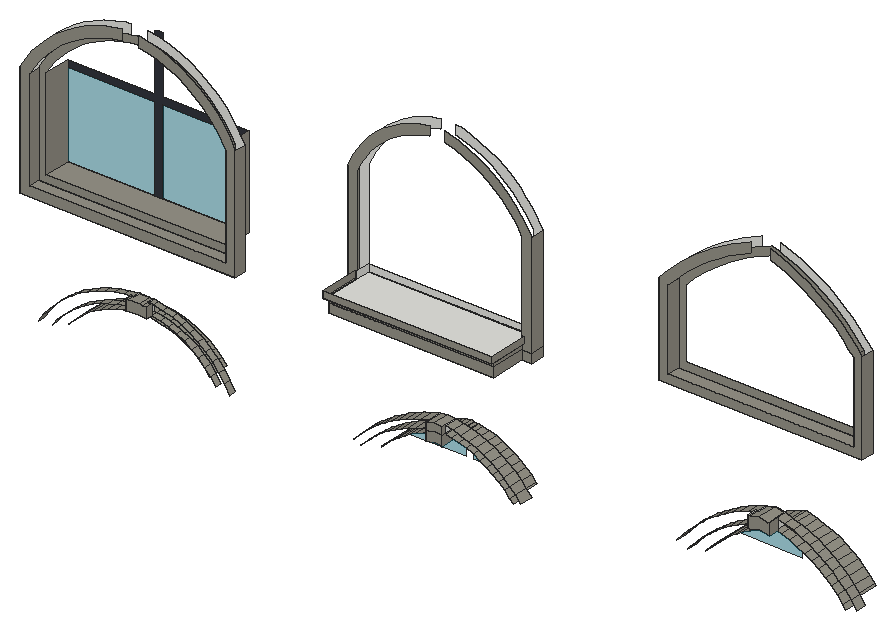
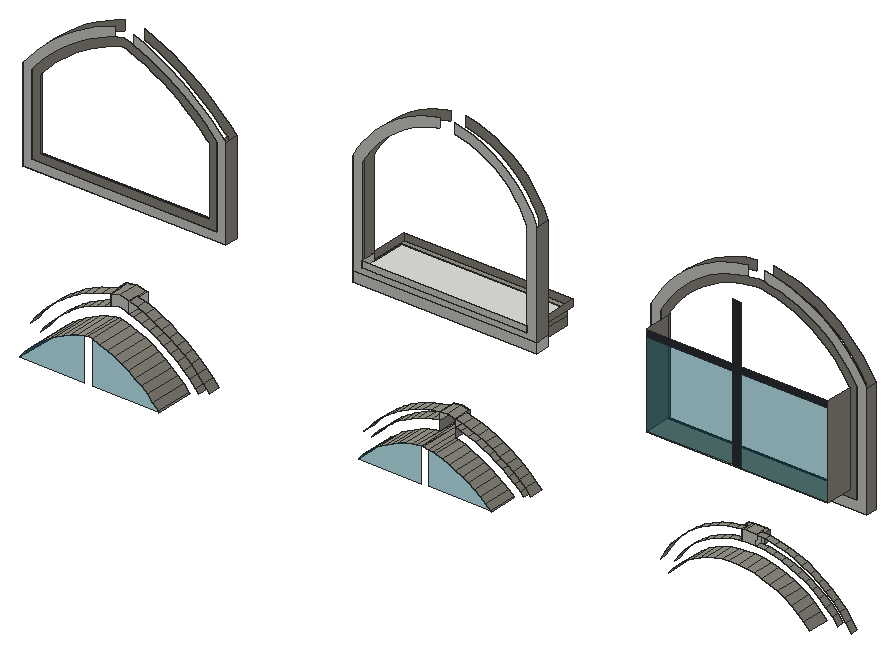
# SketchUp Ruby script. Lengths in inches.
U = 1.inch
M = Sketchup.active_model
def pt(a) = Geom::Point3d.new(a.map { |v| v * U })
def face(e, loops, mat)
  f = e.add_face(loops[0].map { |a| pt(a) })
  loops[1..].each { |l| e.add_face(l.map { |a| pt(a) }).erase! }
  f.material = f.back_material = mat if mat
  f
end
# faces: each face lists its corners as indices into pts; further lists are holes
def faces(e, pts, list, mat = nil) = list.each { |f| face(e, (f[0].is_a?(Array) ? f : [f]).map { |l| l.map { |i| pts[i] } }, mat) }
# xy, xz, yz: faces in a plane at the given z, y or x. An outline is a flat list of corners, or four numbers for a rectangle; further outlines are holes
def ring(l) = l.size == 4 ? [[l[0], l[1]], [l[2], l[1]], [l[2], l[3]], [l[0], l[3]]] : l.each_slice(2).to_a
def flat(e, list, mat, &to3) = list.each { |f| face(e, (f[0].is_a?(Array) ? f : [f]).map { |l| ring(l).map { |u, v| to3.(u, v) } }, mat) }
def xy(e, z, list, mat = nil) = flat(e, list, mat) { |x, y| [x, y, z] }
def xz(e, y, list, mat = nil) = flat(e, list, mat) { |x, z| [x, y, z] }
def yz(e, x, list, mat = nil) = flat(e, list, mat) { |y, z| [x, y, z] }
def lines(e, pts, list) = list.each { |a, b| e.add_line(pt(pts[a]), pt(pts[b])) }
# prism: a flat outline (further loops are holes) pulled along v
def prism(e, loops, v, mat = nil)
  f = face(e, loops, mat); d = Geom::Vector3d.new(v.map { |x| x * U })
  f.pushpull(f.normal.samedirection?(d) ? d.length : -d.length)
end
def box(e, o, s, mat = nil) = prism(e, [[o, [o[0] + s[0], o[1], o[2]], [o[0] + s[0], o[1] + s[1], o[2]], [o[0], o[1] + s[1], o[2]]]], [0, 0, s[2]], mat)
def at(x, y, z, deg = 0) = Geom::Transformation.translation(pt([x, y, z])) * Geom::Transformation.rotation(ORIGIN, Z_AXIS, deg.degrees)
def axes(o, x, y, z) = Geom::Transformation.new([*x, 0, *y, 0, *z, 0, *pt(o).to_a, 1])
def part(name) = M.definitions.add(name)
# library, detail: a bought-in or finely detailed component or shape, given as its bounding box
def library(name, o, s) = part(name).tap { |d| box(d.entities, o, s) }
def detail(e, o, s) = box(e.add_group.entities, o, s)
def put(e, d, t, mat = nil) = e.add_instance(d, t).tap { |i| i.material = mat if mat }
def group(e, t, mat = nil) = e.add_group.tap { |g| g.transformation = t; g.material = mat if mat }.entities
root = M.entities
M.materials.add("[Formica Graystone]").color = [149, 146, 135]
M.materials.add("[Formica Laminate Dark]").color = [50, 53, 60]
M.materials.add("[Translucent Glass Tinted]").color = [4, 106, 127]
M.materials["[Translucent Glass Tinted]"].alpha = 0.48
xy(root,272.42,[[104.39,144.04,108.99,154.66]],"[Formica Graystone]")
xy(root,276.05,[[111.06,137.54,112.68,140.72]],"[Formica Graystone]")
xy(root,276.22,[[104.21,137.54,109.15,144.04]],"[Formica Graystone]")
xy(root,280.43,[[405.62,147.86,406.74,152.99]],"[Formica Graystone]")
xy(root,280.76,[[415.58,147.86,416.39,152.99]],"[Formica Graystone]")
xy(root,281.33,[[111.06,137.54,112.68,140.72]],"[Formica Graystone]")
xy(root,281.47,[[103.95,137.54,109.38,144.04]],"[Formica Graystone]")
xy(root,286.13,[[405.62,147.86,406.74,152.99]],"[Formica Graystone]")
xy(root,286.38,[[415.58,147.86,416.39,152.99]],"[Formica Graystone]")
xy(root,309.5625,[[48.72,138.29,156.59,144.04]])
xy(root,314.51,[[53.67,138.29,151.64,144.04]],"[Formica Graystone]")
xy(root,318.06,[[57.22,144.04,148.1,157.6]],"[Formica Graystone]")
xy(root,323.85,[[218.68,119.22,218.68,136.91,213.99,136.91,213.99,144.04,306.11,144.04,306.11,136.91,301.43,136.91,301.43,119.22]],"[Formica Graystone]")
xy(root,328.26,[[358.05,151.8,459.74,158.3]],"[Formica Graystone]")
xy(root,328.54,[[218.68,119.22,301.43,119.22,301.43,136.91,306.11,136.91,306.11,144.04,213.99,144.04,213.99,136.91,218.68,136.91]])
xy(root,331.48,[[218.68,119.22,301.43,144.04]])
xy(root,331.48,[[217.8,116.35,218.68,136.91],[218.68,116.35,302.43,119.22],[301.43,119.22,302.43,136.91]],"[Formica Graystone]")
xy(root,332.71,[[362.5,151.8,455.3,158.3]],"[Formica Graystone]")
xz(root,116.35,[[217.8,331.48,302.43,334.79]],"[Formica Graystone]")
xz(root,119.22,[[218.68,323.85,301.43,328.54],[218.68,328.54,301.43,331.48]],"[Formica Graystone]")
xz(root,135.35,[[254.54,271.77,256.47,272.28,258.86,272.77,261.26,272.49,262.53,272.25,262.53,277.12,261.98,277.22,258.65,277.61,255.38,276.9375,254.54,276.72],[254.54,276.72,255.38,276.9375,258.65,277.61,261.98,277.22,262.53,277.12,262.53,280.87,258.49,281.34,254.54,280.53]],"[Formica Graystone]")
xz(root,136.91,[[217.8,331.48,218.68,334.79],[301.43,331.48,302.43,334.79]])
xz(root,136.91,[[213.99,323.85,218.68,328.54],[301.43,323.85,306.11,328.54],[213.99,328.54,218.68,328.54,218.68,331.48,217.8,331.48,217.8,334.79,218.68,334.79,218.68,379.39,220.23,382.79,222.51,386.72,225.14,390.41,228.11,393.84,231.39,396.98,234.95,399.79,238.76,402.25,242.79,404.34,246.99,406.05,251.34,407.34,255.1,408.09,255.1,412.87,250.21,411.9,245.4375,410.47,240.82,408.6,236.4,406.31,232.22,403.6,228.31,400.52,224.71,397.08,221.45,393.3125,218.56,389.25,216.07,384.94,213.99,380.42],[301.43,328.54,306.11,328.54,306.11,380.42,303.62,384.61,300.82,388.61,297.72,392.39,294.35,395.92,290.73,399.19,286.86,402.18,282.79,404.87,278.52,407.25,274.09,409.29,269.52,411,264.83,412.37,262.44,412.87,262.44,408.08,263.69,407.82,268.04,406.55,272.29,404.97,276.4,403.07,280.36,400.86,284.14,398.37,287.72,395.59,291.08,392.56,294.21,389.28,297.08,385.78,299.68,382.07,301.43,379.13,301.43,334.79,302.43,334.79,302.43,331.48,301.43,331.48]],"[Formica Graystone]")
xz(root,137.54,[[111.06,276.05,112.68,276.05,112.68,281.33,111.06,281.33,109.38,281.47,103.95,281.47,102.33,281.4,102.59,276.14,104.21,276.22,109.15,276.22]],"[Formica Graystone]")
xz(root,138.29,[[48.72,309.5625,156.59,309.5625,156.59,366.1875,153.85,371.09,150.69,375.74,147.13,380.09,143.21,384.11,138.94,387.77,134.375,391.05,129.53,393.91,124.46,396.33,119.2,398.3,113.78,399.8,108.25,400.8125,108.25,395.78,112.67,394.96,117.67,393.58,122.52,391.77,127.2,389.53,131.67,386.89,135.88,383.875,139.82,380.5,143.4375,376.79,146.72,372.77,149.64,368.49,151.64,364.9,151.64,314.51,53.67,314.51,53.67,364.79,55.75,368.18,58.81,372.37,62.1875,376.29,65.875,379.93,69.84,383.26,74.0625,386.26,78.51,388.91,83.16,391.19,87.98,393.1,92.93,394.6,97.99,395.71,99.89,395.97,99.89,400.96,97.13,400.59,91.68,399.4,86.34,397.78,81.15,395.73,76.15,393.27,71.35,390.41,66.81,387.18,62.54,383.59,58.57,379.67,54.92,375.45,51.64,370.94,48.72,366.1875]],"[Formica Graystone]")
xz(root,140.72,[[111.06,276.05,112.68,276.05,112.68,281.1875,111.06,281.33],[102.59,276.14,104.21,276.22,103.95,281.47,102.33,281.32],[112.68,281.1875,111.06,281.33,112.68,281.33],[102.33,281.32,102.33,281.4,103.95,281.47]])
xz(root,144.04,[[111.06,276.05,109.15,276.22,104.21,276.22,103.95,281.47,109.38,281.47,111.06,281.33],[103.95,281.47,109.38,281.47,108.82,281.52],[48.72,309.5625,48.72,366.1875,51.64,370.94,54.92,375.45,58.57,379.67,62.54,383.59,66.81,387.18,71.35,390.41,76.15,393.27,81.15,395.73,86.34,397.78,91.68,399.4,97.13,400.59,99.89,400.96,99.89,395.97,97.99,395.71,92.93,394.6,87.98,393.1,83.16,391.19,78.51,388.91,74.0625,386.26,69.84,383.26,65.875,379.93,62.1875,376.29,58.81,372.37,55.75,368.18,53.67,364.79,53.67,314.51,151.64,314.51,151.64,364.9,149.64,368.49,146.72,372.77,143.4375,376.79,139.82,380.5,135.88,383.875,131.67,386.89,127.2,389.53,122.52,391.77,117.67,393.58,112.67,394.96,108.25,395.78,108.25,400.8125,113.78,399.8,119.2,398.3,124.46,396.33,129.53,393.91,134.375,391.05,138.94,387.77,143.21,384.11,147.13,380.09,150.69,375.74,153.85,371.09,156.59,366.1875,156.59,309.5625],[213.99,323.85,306.11,328.54],[213.99,328.54,213.99,380.42,216.07,384.94,218.56,389.25,221.45,393.3125,224.71,397.08,228.31,400.52,232.22,403.6,236.4,406.31,240.82,408.6,245.4375,410.47,250.21,411.9,255.1,412.87,255.1,408.09,251.34,407.34,246.99,406.05,242.79,404.34,238.76,402.25,234.95,399.79,231.39,396.98,228.11,393.84,225.14,390.41,222.51,386.72,220.23,382.79,218.68,379.39,218.68,331.48,301.43,331.48,301.43,379.13,299.68,382.07,297.08,385.78,294.21,389.28,291.08,392.56,287.72,395.59,284.14,398.37,280.36,400.86,276.4,403.07,272.29,404.97,268.04,406.55,263.69,407.82,262.44,408.08,262.44,412.87,264.83,412.37,269.52,411,274.09,409.29,278.52,407.25,282.79,404.87,286.86,402.18,290.73,399.19,294.35,395.92,297.72,392.39,300.82,388.61,303.62,384.61,306.11,380.42,306.11,328.54],
  [218.68,331.48,301.43,334.79]])
xz(root,144.04,[[[53.67,314.51,151.64,314.51,151.64,364.9,149.64,368.49,146.72,372.77,143.4375,376.79,139.82,380.5,135.88,383.875,131.67,386.89,127.2,389.53,122.52,391.77,117.67,393.58,112.67,394.96,108.25,395.78,107.57,395.9,102.76,396.35,99.89,395.97,97.99,395.71,92.93,394.6,87.98,393.1,83.16,391.19,78.51,388.91,74.0625,386.26,69.84,383.26,65.875,379.93,62.1875,376.29,58.81,372.37,55.75,368.18,53.67,364.79],[57.22,318.06,57.22,363.79,58.7,366.21,61.59,370.16,64.78,373.87,68.26,377.31,72.01,380.45,76,383.29,80.2,385.79,84.59,387.95,89.14,389.75,93.83,391.17,98.61,392.22,102.83,392.79,107.08,392.39,111.875,391.51,116.57,390.21,121.14,388.5,125.53,386.4,129.73,383.92,133.69,381.08,137.39,377.91,140.79,374.42,143.875,370.65,146.62,366.62,148.1,363.97,148.1,318.06]]],"[Formica Graystone]")
xz(root,147.86,[[405.62,280.43,406.74,280.43,408.25,280.92,411.27,281.7,414.34,281.1,415.58,280.76,416.39,280.76,416.39,286.38,415.58,286.38,411.11,287.27,406.74,286.13,405.62,286.13]],"[Formica Graystone]")
xz(root,151.8,[[358.05,328.26,459.74,328.26,459.74,374.26,456.48,378.3,453.01,382.14,449.33,385.79,445.45,389.23,441.39,392.45,437.15,395.44,432.76,398.19,428.22,400.69,423.55,402.94,418.76,404.93,413.875,406.64,413.875,401.94,417.18,400.78,421.74,398.88,426.18,396.74,430.51,394.36,434.69,391.74,438.73,388.89,442.6,385.83,446.29,382.55,449.8,379.07,453.1,375.41,455.3,372.69,455.3,332.71,362.5,332.71,362.5,372.52,364.75,374.93,368.27,378.41,371.95,381.74,375.76,384.9,379.7,387.91,383.77,390.74,387.95,393.39,392.24,395.87,396.64,398.16,401.12,400.26,404.07,401.49,404.07,406.31,399.32,404.33,394.66,402.14,390.1,399.77,385.65,397.19,381.31,394.4375,377.08,391.5,372.99,388.38,369.03,385.09,365.22,381.64,361.56,378.03,358.05,374.26]],"[Formica Graystone]")
xz(root,152.99,[[405.62,280.43,406.74,280.43,406.74,286.13,405.62,285.77],[415.58,280.76,416.39,280.76,416.39,286.16,415.58,286.38],[405.62,285.77,405.62,286.13,406.74,286.13],[416.39,286.16,415.58,286.38,416.39,286.38]])
xz(root,157.6,[[100.86,318.06,104.96,318.06,104.96,360.43,148.1,360.43,148.1,363.79,104.96,363.79,104.96,392.59,102.83,392.79,100.86,392.22,100.86,363.79,57.22,363.79,57.22,360.43,100.86,360.43]],"[Formica Laminate Dark]")
xz(root,157.6,[[57.22,318.06,100.86,360.43],[104.96,318.06,148.1,360.43]],"[Translucent Glass Tinted]")
xz(root,158.22,[[225.15,255.25,256.47,255.25,256.47,272.28,254.54,271.77,253.01,271.37,249.6,270.28,246.26,269.01,242.99,267.57,239.79,265.95,236.69,264.16,233.69,262.22,230.79,260.12,228.02,257.86,225.36,255.46],[260.2,255.25,291.83,255.25,291.83,255.67,291.37,256.22,288.95,258.74,286.37,261.08,283.63,263.24,280.74,265.21,277.73,266.97,274.61,268.53,271.38,269.86,268.07,270.97,264.69,271.85,262.53,272.25,260.2,272.49]],"[Translucent Glass Tinted]")
xz(root,158.3,[[406.74,280.43,406.74,286.13,411.11,287.27,415.58,286.38,415.58,280.76,414.34,281.1,411.27,281.7,408.25,280.92],[358.05,328.26,358.05,374.26,361.56,378.03,365.22,381.64,369.03,385.09,372.99,388.38,377.08,391.5,381.31,394.4375,385.65,397.19,390.1,399.77,394.66,402.14,399.32,404.33,404.07,406.31,404.07,401.49,401.12,400.26,396.64,398.16,392.24,395.87,387.95,393.39,383.77,390.74,379.7,387.91,375.76,384.9,371.95,381.74,368.27,378.41,364.75,374.93,362.5,372.52,362.5,332.71,455.3,332.71,455.3,372.69,453.1,375.41,449.8,379.07,446.29,382.55,442.6,385.83,438.73,388.89,434.69,391.74,430.51,394.36,426.18,396.74,421.74,398.88,417.18,400.78,413.875,401.94,413.875,406.64,418.76,404.93,423.55,402.94,428.22,400.69,432.76,398.19,437.15,395.44,441.39,392.45,445.45,389.23,449.33,385.79,453.01,382.14,456.48,378.3,459.74,374.26,459.74,328.26]])
xz(root,158.3,[[[362.5,332.71,455.3,332.71,455.3,372.69,453.1,375.41,449.8,379.07,446.29,382.55,442.6,385.83,438.73,388.89,434.69,391.74,430.51,394.36,426.18,396.74,421.74,398.88,417.18,400.78,413.875,401.94,412.52,402.41,409.0625,403.41,405.7,402.17,404.07,401.49,401.12,400.26,396.64,398.16,392.24,395.87,387.95,393.39,383.77,390.74,379.7,387.91,375.76,384.9,371.95,381.74,368.27,378.41,364.75,374.93,362.5,372.52],[366.31,336.52,366.31,371.02,367.48,372.28,370.89,375.64,374.44,378.86,378.13,381.92,381.94,384.83,385.88,387.56,389.92,390.13,394.08,392.53,398.33,394.75,402.67,396.78,407.09,398.63,409.2,399.41,411.36,398.78,415.8125,397.22,420.18,395.41,424.4375,393.36,428.58,391.07,432.58,388.57,436.44,385.84,440.15,382.91,443.68,379.77,447.04,376.44,450.21,372.9375,451.49,371.35,451.49,336.52]]],"[Formica Graystone]")
xz(root,177.43,[[376.19,255.2,409.53,255.2,409.53,276.51,405.77,275.3,402.08,273.88,398.48,272.26,394.97,270.4375,391.58,268.42,388.3,266.21,385.15,263.83,382.14,261.27,379.28,258.54,376.57,255.66],[413.29,255.2,446.03,255.2,446.03,255.53,445.49,256.25,442.98,259.21,440.27,261.98,437.38,264.58,434.32,266.97,431.11,269.15,427.76,271.12,424.29,272.85,420.71,274.35,417.04,275.61,413.29,276.62]],"[Translucent Glass Tinted]")
yz(root,48.72,[[138.29,309.5625,144.04,366.1875]],"[Formica Graystone]")
yz(root,53.67,[[138.29,314.51,144.04,364.79]],"[Formica Graystone]")
yz(root,57.22,[[144.04,318.06,157.6,363.79]],"[Formica Graystone]")
yz(root,111.06,[[140.72,276.05,144.04,281.33]])
yz(root,112.68,[[137.54,276.05,140.72,281.33]],"[Formica Graystone]")
yz(root,148.1,[[144.04,318.06,157.6,363.97]],"[Formica Graystone]")
yz(root,151.64,[[138.29,314.51,144.04,364.9]],"[Formica Graystone]")
yz(root,156.59,[[138.29,309.5625,144.04,366.1875]],"[Formica Graystone]")
yz(root,213.99,[[136.91,323.85,144.04,328.54]])
yz(root,213.99,[[136.91,328.54,144.04,380.42]],"[Formica Graystone]")
yz(root,217.8,[[116.35,331.48,136.91,334.79]],"[Formica Graystone]")
yz(root,218.68,[[136.91,331.48,144.04,334.79]])
yz(root,218.68,[[119.22,323.85,136.91,328.54],[119.22,328.54,136.91,331.48]],"[Formica Graystone]")
yz(root,254.54,[[137.35,276.72,144.04,280.53]])
yz(root,254.54,[[135.35,271.77,144.04,276.72],[135.35,276.72,137.35,280.53]],"[Formica Graystone]")
yz(root,262.53,[[137.35,277.12,144.04,280.87]])
yz(root,262.53,[[135.35,272.25,144.04,277.12],[135.35,277.12,137.35,280.87]],"[Formica Graystone]")
yz(root,301.43,[[136.91,331.48,144.04,334.79]])
yz(root,301.43,[[119.22,323.85,136.91,328.54],[119.22,328.54,136.91,331.48]],"[Formica Graystone]")
yz(root,302.43,[[116.35,331.48,136.91,334.79]],"[Formica Graystone]")
yz(root,306.11,[[136.91,323.85,144.04,328.54],[136.91,328.54,144.04,380.42]],"[Formica Graystone]")
yz(root,358.05,[[151.8,328.26,158.3,374.26]],"[Formica Graystone]")
yz(root,362.5,[[151.8,332.71,158.3,372.52]],"[Formica Graystone]")
yz(root,405.62,[[147.86,280.43,152.99,286.13]])
yz(root,406.74,[[152.99,280.43,158.3,286.13]])
yz(root,415.58,[[152.99,280.76,158.3,286.38]])
yz(root,416.39,[[147.86,280.76,152.99,286.38]],"[Formica Graystone]")
yz(root,455.3,[[151.8,332.71,158.3,372.69]],"[Formica Graystone]")
yz(root,459.74,[[151.8,328.26,158.3,374.26]],"[Formica Graystone]")
p = [[58.9375,144.04,257.72],[56.17,144.04,253.84],[56.17,140.72,253.84],[58.9375,140.72,257.72],[151.73,144.04,253.84],[149.35,144.04,258.08],
  [149.35,140.72,258.08],[151.73,140.72,253.84],[63.1,144.04,254.5],[65.9,144.04,257.84],[65.9,140.72,257.84],[63.1,140.72,254.5],
  [225.36,144.04,255.46],[225.15,144.04,255.25],[225.15,158.22,255.25],[225.36,158.22,255.46],[376.57,158.3,255.66],[376.19,158.3,255.2],
  [376.19,177.43,255.2],[376.57,177.43,255.66],[142.4,144.04,258.86],[144.89,144.04,255.28],[144.89,140.72,255.28],[142.4,140.72,258.86],
  [71.5625,144.04,258.2],[68.72,144.04,255.29],[68.72,154.66,255.29],[71.5625,154.66,258.2],[228.02,144.04,257.86],[228.02,158.22,257.86],
  [446.03,158.3,255.53],[445.49,158.3,256.25],[445.49,177.43,256.25],[446.03,177.43,255.53],[291.83,144.04,255.67],[291.37,144.04,256.22],
  [291.37,158.22,256.22],[291.83,158.22,255.67],[379.28,158.3,258.54],[379.28,177.43,258.54],[288.95,144.04,258.74],[288.95,158.22,258.74],
  [442.98,158.3,259.21],[442.98,177.43,259.21],[139.39,144.04,256.53],[136.8,144.04,259.57],[136.8,154.66,259.57],[139.39,154.66,256.53],
  [371.6,158.3,256.87],[373.14,158.3,258.7],[373.14,152.99,258.7],[371.6,152.99,256.87],[449.09,158.3,259.11],[450.625,158.3,257.05],
  [450.625,152.99,257.05],[449.09,152.99,259.11],[220.36,144.04,257.22],[222.06,144.04,258.93],[222.06,137.35,258.93],[220.36,137.35,257.22],
  [294.9375,144.04,259.41],[296.61,144.04,257.41],[296.61,137.35,257.41],[294.9375,137.35,259.41],[62,144.04,261.375],[62,140.72,261.375],
  [68.95,144.04,260.96],[68.95,140.72,260.96],[230.79,144.04,260.12],[230.79,158.22,260.12],[146.5625,144.04,262.07],[146.5625,140.72,262.07],
  [74.62,144.04,260.875],[74.62,154.66,260.875],[382.14,158.3,261.27],[382.14,177.43,261.27],[219.52,144.04,261.6],[216.67,144.04,258.75],
  [216.67,137.35,258.75],[219.52,137.35,261.6],[300.3,144.04,258.75],[297.68,144.04,261.875],[297.68,137.35,261.875],[300.3,137.35,258.75],
  [286.37,144.04,261.08],[286.37,158.22,261.08],[376.02,158.3,261.77],[376.02,152.99,261.77],[369.07,158.3,262.3],[366.17,158.3,258.84],
  [366.17,152.99,258.84],[369.07,152.99,262.3],[456.05,158.3,258.84],[453.33,158.3,262.49],[453.33,152.99,262.49],[456.05,152.99,258.84],
  [224.9,144.04,261.5],[224.9,137.35,261.5],[139.57,144.04,262.17],[139.57,140.72,262.17],[446.37,158.3,262.3],[446.37,152.99,262.3],
  [440.27,158.3,261.98],[440.27,177.43,261.98],[292.29,144.04,262.17],[292.29,137.35,262.17],[133.93,144.04,262.34],[133.93,154.66,262.34],
  [233.69,144.04,262.22],[233.69,158.22,262.22],[77.88,144.04,263.31],[77.88,154.66,263.31],[72.23,144.04,263.83],[72.23,140.72,263.83],
  [283.63,144.04,263.24],[283.63,158.22,263.24],[385.15,158.3,263.83],[385.15,177.43,263.83],[65.34,144.04,264.78],[65.34,140.72,264.78],
  [227.88,144.04,263.91],[227.88,137.35,263.91],[222.51,144.04,264.3],[222.51,137.35,264.3],[379.0625,158.3,264.68],[379.0625,152.99,264.68],
  [294.86,144.04,264.8125],[294.86,137.35,264.8125],[437.38,158.3,264.58],[437.38,177.43,264.58],[143.4,144.04,265.78],[143.4,140.72,265.78],
  [289.46,144.04,264.73],[289.46,137.35,264.73],[136.43,144.04,265.2],[136.43,140.72,265.2],[236.69,144.04,264.16],[236.69,158.22,264.16],
  [130.8,144.04,264.82],[130.8,154.66,264.82],[372.16,158.3,265.6],[372.16,152.99,265.6],[443.45,158.3,265.3],[443.45,152.99,265.3],
  [450.38,158.3,265.96],[450.38,152.99,265.96],[280.74,144.04,265.21],[280.74,158.22,265.21],[81.32,144.04,265.48],[81.32,154.66,265.48],
  [75.73,144.04,266.4375],[75.73,140.72,266.4375],[388.3,158.3,266.21],[388.3,177.43,266.21],[230.98,144.04,266.16],[230.98,137.35,266.16],
  [239.79,144.04,265.95],[239.79,158.22,265.95],[225.63,144.04,266.84],[225.63,137.35,266.84],[434.32,158.3,266.97],[434.32,177.43,266.97],
  [286.46,144.04,267.1],[286.46,137.35,267.1],[382.27,158.3,267.41],[382.27,152.99,267.41],[291.84,144.04,267.55],[291.84,137.35,267.55],
  [68.93,144.04,267.92],[68.93,140.72,267.92],[127.45,144.04,266.98],[127.45,154.66,266.98],[133.02,144.04,267.9],[133.02,140.72,267.9],
  [277.73,144.04,266.97],[277.73,158.22,266.97],[440.33,158.3,268.1],[440.33,152.99,268.1],[84.92,144.04,267.375],[84.92,154.66,267.375],
  [375.43,158.3,268.71],[375.43,152.99,268.71],[139.9,144.04,269.16],[139.9,140.72,269.16],[242.99,144.04,267.57],[242.99,158.22,267.57],
  [447.21,158.3,269.22],[447.21,152.99,269.22],[234.2,144.04,268.25],[234.2,137.35,268.25],[391.58,158.3,268.42],[391.58,177.43,268.42],
  [79.42,144.04,268.77],[79.42,140.72,268.77],[228.89,144.04,269.21],[228.89,137.35,269.21],[123.91,144.04,268.81],[123.91,154.66,268.81],
  [274.61,144.04,268.53],[274.61,158.22,268.53],[431.11,158.3,269.15],[431.11,177.43,269.15],[283.3,144.04,269.25],[283.3,137.35,269.25],
  [88.65,144.04,268.99],[88.65,154.66,268.99],[385.625,158.3,269.95],[385.625,152.99,269.95],[288.64,144.04,270.08],[288.64,137.35,270.08],
  [246.26,144.04,269.01],[246.26,158.22,269.01],[72.75,144.04,270.78],[72.75,140.72,270.78],[129.35,144.04,270.27],[129.35,140.72,270.27],
  [437.03,158.3,270.68],[437.03,152.99,270.68],[237.52,144.04,270.16],[237.52,137.35,270.16],[394.97,158.3,270.4375],[394.97,177.43,270.4375],
  [271.38,144.04,269.86],[271.38,158.22,269.86],[378.87,158.3,271.64],[378.87,152.99,271.64],[83.27,144.04,270.8],[83.27,140.72,270.8],
  [120.2,144.04,270.28],[120.2,154.66,270.28],[92.49,144.04,270.31],[92.49,154.66,270.31],[249.6,144.04,270.28],[249.6,158.22,270.28],
  [232.27,144.04,271.4],[232.27,137.35,271.4],[136.08,144.04,272.18],[136.08,140.72,272.18],[443.82,158.3,272.26],[443.82,152.99,272.26],
  [427.76,158.3,271.12],[427.76,177.43,271.12],[280.01,144.04,271.19],[280.01,137.35,271.19],[268.07,144.04,270.97],[268.07,158.22,270.97],
  [389.12,158.3,272.3],[389.12,152.99,272.3],[285.28,144.04,272.37],[285.28,137.35,272.37],[240.9375,144.04,271.89],[240.9375,137.35,271.89],
  [125.48,144.04,272.26],[125.48,140.72,272.26],[96.43,144.04,271.33],[96.43,154.66,271.33],[116.37,144.04,271.39],[116.37,154.66,271.39],
  [253.01,144.04,271.37],[253.01,158.22,271.37],[398.48,158.3,272.26],[398.48,177.43,272.26],[433.57,158.3,273.04],[433.57,152.99,273.04],
  [76.78,144.04,273.32],[76.78,140.72,273.32],[87.28,144.04,272.53],[87.28,140.72,272.53],[264.69,144.04,271.85],[264.69,158.22,271.85],
  [424.29,158.3,272.85],[424.29,177.43,272.85],[276.59,144.04,272.88],[276.59,137.35,272.88],[100.4375,144.04,272.03],[100.4375,154.66,272.03],
  [235.76,144.04,273.4],[235.76,137.35,273.4],[112.45,144.04,272.12],[112.45,154.66,272.12],[254.54,144.04,271.77],[254.54,158.22,271.77],
  [382.47,158.3,274.37],[382.47,152.99,274.37],[256.47,158.22,272.28],[256.47,135.35,272.28],[254.54,135.35,271.77],[262.53,158.22,272.25],
  [262.53,144.04,272.25],[244.44,144.04,273.4375],[244.44,137.35,273.4375],[104.39,144.04,272.42],[104.39,154.66,272.42],[108.99,144.04,272.42],
  [108.99,154.66,272.42],[131.99,144.04,274.82],[131.99,140.72,274.82],[258.86,158.22,272.77],[258.86,135.35,272.77],[260.2,158.22,272.49],
  [261.26,135.35,272.49],[262.53,135.35,272.25],[121.43,144.04,273.875],[121.43,140.72,273.875],[392.74,158.3,274.45],[392.74,152.99,274.45],
  [440.23,158.3,275.0625],[440.23,152.99,275.0625],[402.08,158.3,273.88],[402.08,177.43,273.88],[281.76,144.04,274.43],[281.76,137.35,274.43],
  [91.4,144.04,273.95],[91.4,140.72,273.95],[273.06,144.04,274.34],[273.06,137.35,274.34],[420.71,158.3,274.35],[420.71,177.43,274.35],
  [429.96,158.3,275.16],[429.96,152.99,275.16],[81,144.04,275.55],[81,140.72,275.55],[239.36,144.04,275.22],[239.36,137.35,275.22],
  [248.03,144.04,274.8],[248.03,137.35,274.8],[95.625,144.04,275.04],[95.625,140.72,275.04],[117.24,144.04,275.09],[117.24,140.72,275.09],
  [405.77,158.3,275.3],[405.77,177.43,275.3],[269.43,144.04,275.56],[269.43,137.35,275.56],[278.11,144.04,276.24],[278.11,137.35,276.24],
  [386.22,158.3,276.89],[386.22,152.99,276.89],[417.04,158.3,275.61],[417.04,177.43,275.61],[396.48,158.3,276.39],[396.48,152.99,276.39],
  [251.68,144.04,275.97],[251.68,137.35,275.97],[127.66,144.04,277.06],[127.66,140.72,277.06],[99.92,144.04,275.8],[99.92,140.72,275.8],
  [112.96,144.04,275.88],[112.96,140.72,275.88],[436.47,158.3,277.625],[436.47,152.99,277.625],[243.04,144.04,276.85],[243.04,137.35,276.85],
  [426.21,158.3,277.03],[426.21,152.99,277.03],[409.53,158.3,276.51],[409.53,177.43,276.51],[85.38,144.04,277.44],[85.38,140.72,277.44],
  [265.73,144.04,276.52],[265.73,137.35,276.52],[413.29,158.3,276.62],[413.29,177.43,276.62],[104.21,144.04,276.22],[104.21,140.72,276.22],
  [111.06,144.04,276.05],[111.06,140.72,276.05],[254.54,144.04,276.72],[254.54,137.35,276.72],[102.33,137.54,281.4],[102.33,140.72,281.4],
  [102.33,140.72,281.32],[102.59,140.72,276.14],[102.59,137.54,276.14],[104.21,137.54,276.22],[109.15,144.04,276.22],[111.06,137.54,276.05],
  [109.15,137.54,276.22],[274.35,144.04,277.8],[274.35,137.35,277.8],[103.95,144.04,281.47],[103.95,140.72,281.47],[400.3125,158.3,278.12],
  [400.3125,152.99,278.12],[262.53,144.04,277.12],[262.53,137.35,277.12],[411.41,158.3,277],[411.41,177.43,277],[246.81,144.04,278.28],
  [246.81,137.35,278.28],[390.1,158.3,279.19],[390.1,152.99,279.19],[422.35,158.3,278.65],[422.35,152.99,278.65],[123.14,144.04,278.86],
  [123.14,140.72,278.86],[89.89,144.04,278.99],[89.89,140.72,278.99],[432.55,158.3,279.93],[432.55,152.99,279.93],[270.48,144.04,279.1],
  [270.48,137.35,279.1],[404.24,158.3,279.63],[404.24,152.99,279.63],[250.64,144.04,279.51],[250.64,137.35,279.51],[418.38,158.3,280.01],
  [418.38,152.99,280.01],[118.46,144.04,280.21],[118.46,140.72,280.21],[94.51,144.04,280.18],[94.51,140.72,280.18],[266.54,144.04,280.12],
  [266.54,137.35,280.12],[394.11,158.3,281.28],[394.11,152.99,281.28],[254.54,144.04,280.53],[254.54,137.35,280.53],[406.74,158.3,280.43],
  [406.74,152.99,280.43],[428.47,158.3,281.96],[428.47,152.99,281.96],[415.58,158.3,280.76],[415.58,152.99,280.76],[262.53,144.04,280.87],
  [262.53,137.35,280.87],[99.21,144.04,281.01],[99.21,140.72,281.01],[113.67,144.04,281.1],[113.67,140.72,281.1],[408.25,158.3,280.92],
  [408.25,147.86,280.92],[406.74,147.86,280.43],[258.49,144.04,281.34],[254.54,135.35,280.53],[258.49,135.35,281.34],[414.34,158.3,281.1],
  [415.58,147.86,280.76],[414.34,147.86,281.1],[262.53,135.35,280.87],[411.27,158.3,281.7],[411.27,147.86,281.7],[111.06,144.04,281.33],
  [111.06,140.72,281.33],[112.68,140.72,281.1875],[109.38,144.04,281.47],[109.38,137.54,281.47],[111.06,137.54,281.33],[398.22,158.3,283.13],
  [398.22,152.99,283.13],[103.95,137.54,281.47],[424.28,158.3,283.72],[424.28,152.99,283.72],[402.44,158.3,284.75],[402.44,152.99,284.75],
  [419.97,158.3,285.2],[419.97,152.99,285.2],[406.74,158.3,286.13],[405.62,152.99,285.77],[406.74,152.99,286.13],[415.58,158.3,286.38],
  [415.58,152.99,286.38],[416.39,152.99,286.16],[411.11,158.3,287.27],[406.74,147.86,286.13],[411.11,147.86,287.27],[415.58,147.86,286.38]]
faces(root,p,[[0,1,2,3],[4,5,6,7],[8,9,10,11],[12,13,14,15],[16,17,18,19],[20,21,22,23],[24,25,26,27],[28,12,15,29],
  [30,31,32,33],[34,35,36,37],[38,16,19,39],[35,40,41,36],[31,42,43,32],[44,45,46,47],[48,49,50,51],[52,53,54,55],
  [56,57,58,59],[60,61,62,63],[64,0,3,65],[9,66,67,10],[68,28,29,69],[5,70,71,6],[72,24,27,73],[74,38,39,75],
  [76,77,78,79],[80,81,82,83],[40,84,85,41],[49,86,87,50],[88,89,90,91],[92,93,94,95],[57,96,97,58],[98,20,23,99],
  [100,52,55,101],[42,102,103,43],[104,60,63,105],[45,106,107,46],[108,68,69,109],[110,72,73,111],[66,112,113,67],[84,114,115,85],
  [116,74,75,117],[118,64,65,119],[96,120,121,97],[122,76,79,123],[86,124,125,87],[81,126,127,82],[102,128,129,103],[70,130,131,71],
  [132,104,105,133],[134,98,99,135],[136,108,109,137],[106,138,139,107],[140,88,91,141],[142,100,101,143],[93,144,145,94],[114,146,147,115],
  [148,110,111,149],[112,150,151,113],[152,116,117,153],[120,154,155,121],[156,136,137,157],[158,122,123,159],[128,160,161,129],[162,132,133,163],
  [124,164,165,125],[126,166,167,127],[168,118,119,169],[138,170,171,139],[172,134,135,173],[146,174,175,147],[176,142,143,177],[178,148,149,179],
  [180,140,141,181],[130,182,183,131],[184,156,157,185],[144,186,187,145],[154,188,189,155],[190,152,153,191],[150,192,193,151],[194,158,159,195],
  [170,196,197,171],[174,198,199,175],[160,200,201,161],[202,162,163,203],[204,178,179,205],[164,206,207,165],[166,208,209,167],[210,184,185,211],
  [212,168,169,213],[214,172,173,215],[216,176,177,217],[188,218,219,189],[220,190,191,221],[198,222,223,199],[224,180,181,225],[192,226,227,193],
  [196,228,229,197],[230,204,205,231],[232,210,211,233],[234,194,195,235],[182,236,237,183],[186,238,239,187],[200,240,241,201],[242,202,203,243],
  [222,244,245,223],[206,246,247,207],[208,248,249,209],[218,250,251,219],[252,214,215,253],[254,230,231,255],[228,256,257,229],[258,232,233,259],
  [260,220,221,261],[262,216,217,263],[264,212,213,265],[226,266,267,227],[244,268,269,245],[240,270,271,241],[272,242,243,273],[274,254,255,275],
  [276,234,235,277],[256,278,279,257],[280,258,259,281],[282,224,225,283],[284,285,286,280,281],[287,269,268,288],[250,289,290,251],[291,274,275,292],
  [278,293,294,279],[236,295,296,237],[284,297,298,285],[299,287,300],[300,287,288,301],[302,252,253,303],[246,304,305,247],[238,306,307,239],
  [308,260,261,309],[248,310,311,249],[297,299,298],[300,298,299],[266,312,313,267],[314,272,273,315],[270,316,317,271],[318,262,263,319],
  [320,264,265,321],[322,276,277,323],[289,324,325,290],[312,326,327,313],[328,302,303,329],[330,308,309,331],[332,314,315,333],[310,334,335,311],
  [336,282,283,337],[316,338,339,317],[304,340,341,305],[324,342,343,325],[295,344,345,296],[326,346,347,327],[348,328,329,349],[306,350,351,307],
  [352,322,323,353],[354,318,319,355],[356,330,331,357],[358,320,321,359],[360,332,333,361],[338,362,363,339],[346,364,365,347],[366,348,349,367],
  [342,368,369,343],[370,371,372,373,374],[365,375,374,373],[376,366,367,377,378],[334,379,380,335],[340,383,384,341],[385,360,361,386],[387,356,357,388],
  [362,387,388,363],[389,352,353,390],[391,336,337,392],[393,354,355,394],[344,395,396,345],[397,358,359,398],[350,399,400,351],[379,401,402,380],
  [383,403,404,384],[405,389,390,406],[407,393,394,408],[395,409,410,396],[411,397,398,412],[401,413,414,402],[415,391,392,416],[417,405,406,418],
  [403,419,420,404],[399,421,422,400],[423,407,408,424],[413,425,426,414],[427,411,412,428],[409,429,430,410],[419,431,432,433,420],[434,417,418,435,436],
  [437,423,424,438,439],[425,434,436,440,426],[431,441,442,432],[381,427,428,372,382],[429,443,444,445,430],[441,437,439,442],[443,446,447,448,444],[449,415,416,450],
  [451,382,371,370],[421,452,453,422],[454,449,450,455],[452,456,457,453],[458,454,455,459,460],[456,461,462,463,457],[464,458,460,465,466],[461,464,466,467,462]],"[Formica Graystone]")
faces(root,p,[[381,364,365,382]])
